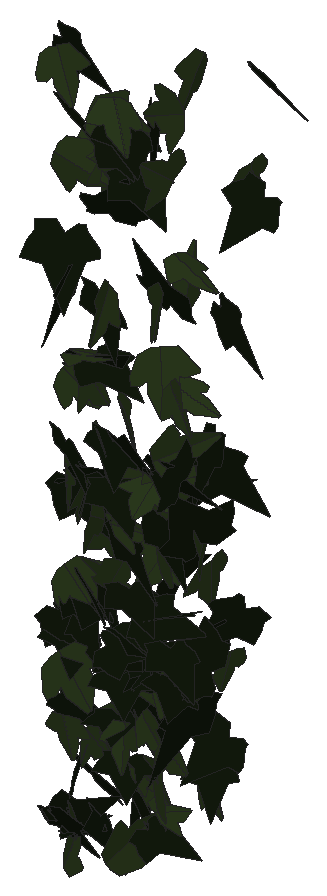
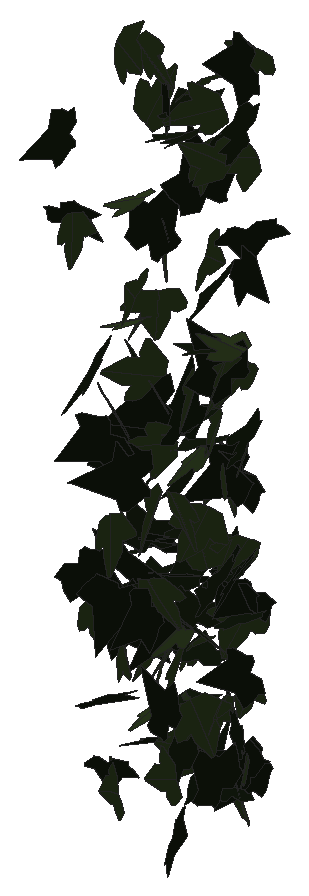
# SketchUp Ruby script. Lengths in inches.
U = 1.inch
M = Sketchup.active_model
def pt(a) = Geom::Point3d.new(a.map { |v| v * U })
def face(e, loops, mat)
  f = e.add_face(loops[0].map { |a| pt(a) })
  loops[1..].each { |l| e.add_face(l.map { |a| pt(a) }).erase! }
  f.material = f.back_material = mat if mat
  f
end
# faces: each face lists its corners as indices into pts; further lists are holes
def faces(e, pts, list, mat = nil) = list.each { |f| face(e, (f[0].is_a?(Array) ? f : [f]).map { |l| l.map { |i| pts[i] } }, mat) }
# xy, xz, yz: faces in a plane at the given z, y or x. An outline is a flat list of corners, or four numbers for a rectangle; further outlines are holes
def ring(l) = l.size == 4 ? [[l[0], l[1]], [l[2], l[1]], [l[2], l[3]], [l[0], l[3]]] : l.each_slice(2).to_a
def flat(e, list, mat, &to3) = list.each { |f| face(e, (f[0].is_a?(Array) ? f : [f]).map { |l| ring(l).map { |u, v| to3.(u, v) } }, mat) }
def xy(e, z, list, mat = nil) = flat(e, list, mat) { |x, y| [x, y, z] }
def xz(e, y, list, mat = nil) = flat(e, list, mat) { |x, z| [x, y, z] }
def yz(e, x, list, mat = nil) = flat(e, list, mat) { |y, z| [x, y, z] }
def lines(e, pts, list) = list.each { |a, b| e.add_line(pt(pts[a]), pt(pts[b])) }
# prism: a flat outline (further loops are holes) pulled along v
def prism(e, loops, v, mat = nil)
  f = face(e, loops, mat); d = Geom::Vector3d.new(v.map { |x| x * U })
  f.pushpull(f.normal.samedirection?(d) ? d.length : -d.length)
end
def box(e, o, s, mat = nil) = prism(e, [[o, [o[0] + s[0], o[1], o[2]], [o[0] + s[0], o[1] + s[1], o[2]], [o[0], o[1] + s[1], o[2]]]], [0, 0, s[2]], mat)
def at(x, y, z, deg = 0) = Geom::Transformation.translation(pt([x, y, z])) * Geom::Transformation.rotation(ORIGIN, Z_AXIS, deg.degrees)
def axes(o, x, y, z) = Geom::Transformation.new([*x, 0, *y, 0, *z, 0, *pt(o).to_a, 1])
def part(name) = M.definitions.add(name)
# library, detail: a bought-in or finely detailed component or shape, given as its bounding box
def library(name, o, s) = part(name).tap { |d| box(d.entities, o, s) }
def detail(e, o, s) = box(e.add_group.entities, o, s)
def put(e, d, t, mat = nil) = e.add_instance(d, t).tap { |i| i.material = mat if mat }
def group(e, t, mat = nil) = e.add_group.tap { |g| g.transformation = t; g.material = mat if mat }.entities
root = M.entities
M.materials.add("efeu1").color = [18, 25, 13]
M.materials.add("efeu2").color = [43, 57, 29]
c1 = part("ivyleaf_9")
p = [[1.54,2.16,1.25],[1.36,2.04,1.19],[-0.21,0.99,0.68],[-0.71,1.11,0.82],[-0.85,0.86,0.67],[-0.8,0.17,0.21],
  [-0.9,-0.01,0.1],[-0.67,-0.16,-0.02],[-0.08,-0.08,-0.05],[-0.03,-0.6,-0.4],[0.65,-0.88,-0.66],[0.83,-0.6,-0.49],
  [1.29,-0.42,-0.43],[1.8125,-0.07,-0.26],[1.21,0.44,0.15]]
faces(c1.entities,p,[[0,1,2,3,4,5,6,7,8,9,10,11,12,13,14]],"efeu1")
c2 = part("ivyleaf_10")
p = [[0,0.5,-0.03],[-0.0625,2.02,-0.43],[-0.19,2.01,-0.46],[-0.54,1.05,-0.29],[-0.52,0.625,-0.18],[-0.83,0.76,-0.28],
  [-1.16,0.64,-0.33],[-1.15,0.33,-0.24],[-0.77,-0.39,0.02],[-0.3,-0.51,0.16],[0.04,-0.48,0.23],[-0.02,2.01,-0.4375],
  [-0.06,2.01,-0.43],[0.04,-0.49,0.23],[0.67,-0.49,0.14],[1.38,0.36,-0.2],[1.375,0.51,-0.24],[0.81,0.65,-0.19],
  [0.62,0.59,-0.15],[0.6,1.09,-0.28],[0.5,1.23,-0.31]]
faces(c2.entities,p,[[0,1,2,3,4,5,6,7,8,9,10],[11,12,0,13,14,15,16,17,18,19,20]],"efeu2")
put(root,c1,axes([585.51,133.55,206.23],[0.0501,-0.05438,-1.04227],[0.86065,-0.58813,0.07206],[-0.5904,-0.86195,0.0166]))
put(root,c2,axes([585.95,127.96,211.29],[-0.83136,-0.03017,-0.08429],[0.08725,-0.09703,-0.82592],[0.02002,-0.82997,0.09962]))
put(root,c1,axes([585.42,128.3,216.13],[-0.09026,-0.32634,-0.83286],[0.52136,0.66101,-0.31551],[0.72686,-0.51465,0.12288]))
put(root,c2,axes([585.97,128.1,207.37],[-0.60504,0.54503,-0.03185],[0.01034,-0.03609,-0.81409],[-0.54586,-0.6048,0.01987]))
put(root,c1,axes([585.38,128.72,223.79],[0.42595,-0.76263,0.4513],[0.2309,-0.38792,-0.87346],[0.85555,0.48439,0.01104]))
put(root,c1,axes([585.28,128.95,239.36],[0.80558,-0.65014,0.25019],[0.21213,-0.13539,-1.03485],[0.66354,0.8326,0.02708]))
put(root,c1,axes([585.71,128.67,217.36],[0.49087,-0.72835,-0.41678],[-0.24025,0.34065,-0.87828],[0.80403,0.54645,-0.00799]))
put(root,c2,axes([585.78,128.51,227.15],[0.23963,0.72854,0.60869],[0.14768,0.59153,-0.76615],[-0.9378,0.27931,0.03489]))
put(root,c1,axes([585.8,128.06,233.9],[-0.38131,-0.98409,-0.33251],[0.16177,0.29362,-1.05452],[1.02607,-0.412,0.04269]))
put(root,c1,axes([585.67,128.77,214.84],[-0.23101,-0.84302,0.2977],[0.43214,-0.37446,-0.72505],[0.78266,-0.04207,0.48821]))
put(root,c2,axes([585.89,128.11,223.14],[-0.28014,0.63865,-0.5658],[0.20325,-0.52843,-0.6971],[-0.82868,-0.34551,0.02029]))
put(root,c1,axes([585.73,127.48,207.18],[0.96679,0.0946,-0.04957],[-0.04934,-0.00483,-0.97141],[-0.09472,0.96805,-0.00001]))
put(root,c1,axes([585.28,128.7,242.55],[0.21299,0.05407,-1.0631],[1.01754,0.30807,0.21953],[0.31262,-1.03954,0.00976]))
put(root,c1,axes([585.35,130.5,207.51],[0.24464,-0.58363,0.86638],[0.69801,-0.5707,-0.58154],[0.77719,0.69626,0.24958]))
put(root,c2,axes([586.21,128.98,222.03],[0.28492,-0.90487,-0.01439],[-0.00315,0.0141,-0.94866],[0.90498,0.28494,0.00123]))
put(root,c1,axes([585.48,128.43,212.1875],[0.11884,0.08634,-0.90899],[0.69514,0.5858,0.14653],[0.59204,-0.70515,0.01043]))
put(root,c1,axes([586.16,127.97,232.18],[-0.42791,0.42905,-0.87197],[0.63431,-0.5985,-0.60578],[-0.73625,-0.76501,-0.01511]))
put(root,c2,axes([585.98,128.12,204.92],[0.71411,-0.50695,-0.16028],[0.13019,-0.0935,0.87575],[-0.5155,-0.72588,-0.00086]))
put(root,c1,axes([585.99,128.37,208.41],[-0.04442,0.59072,0.69736],[0.04222,-0.69611,0.59235],[0.91295,0.06093,0.00654]))
put(root,c1,axes([585.72,128.72,222.29],[0.86826,0.29098,0.41673],[0.39648,0.12836,-0.91571],[-0.31801,0.95449,-0.0039]))
put(root,c2,axes([585.89,127.55,242.44],[0.86652,0.24684,0.42001],[0.40095,0.12548,-0.90094],[-0.27673,0.95473,0.00981]))
put(root,c2,axes([586.05,128.14,218.14],[0.3506,0.79192,0.47898],[0.19955,0.43547,-0.86604],[-0.90374,0.40338,-0.00541]))
put(root,c1,axes([585.67,128.7,222.19],[-0.13848,-0.22747,-1.05466],[0.8716,0.60312,-0.24453],[0.6359,-0.87621,0.10548]))
put(root,c2,axes([586.7,130.58,210.77],[-0.50125,-0.91522,0.38623],[-0.16473,-0.35004,-1.04326],[0.97963,-0.52716,0.02219]))
put(root,c1,axes([585.875,127.98,206.74],[0.09236,-0.0552,0.89328],[0.8896,0.104,-0.08555],[-0.09801,0.892,0.06525]))
put(root,c2,axes([586.33,128.9375,227.13],[0.23077,-0.84715,-0.50017],[0.28382,0.54923,-0.7993],[0.94195,0.04205,0.36337]))
put(root,c1,axes([586.02,128.57,216.49],[-0.32118,-0.34753,-0.79455],[0.69984,0.39652,-0.45633],[0.51216,-0.75976,0.12528]))
put(root,c2,axes([586.39,128.93,210.46],[0.20739,-0.73113,-0.50407],[0.25485,0.54486,-0.68544],[0.8507,0.01501,0.32823]))
put(root,c1,axes([585.88,130.07,217.07],[0.50797,-0.90302,0.37203],[0.18325,-0.32377,-1.03609],[0.95931,0.54001,0.00092]))
put(root,c2,axes([585.87,128.15,237.55],[-0.37364,-0.05689,-1.03887],[1.03345,-0.14794,-0.36359],[-0.12031,-1.09407,0.10319]))
put(root,c1,axes([586.04,128.92,206.21],[0.07892,-0.79624,0.09225],[0.78778,0.05993,-0.15666],[0.14801,0.10558,0.78465]))
put(root,c1,axes([585.93,129.24,227.16],[0.96059,0.40208,-0.31312],[0.29049,0.11694,1.04134],[0.41872,-1.00355,-0.00411]))
put(root,c1,axes([586.33,129.03,216.81],[-0.25324,-0.72445,0.51195],[0.3658,-0.57031,-0.62608],[0.80815,0.03113,0.44381]))
put(root,c2,axes([586.91,131.49,221.44],[0.88052,-0.45234,-0.39639],[-0.34182,0.20187,-0.98968],[0.49486,0.9443,0.02169]))
put(root,c2,axes([586.375,127.38,214.44],[0.58733,0.8968,0.53146],[0.18045,0.51333,-1.06564],[-1.02671,0.60323,0.11673]))
put(root,c2,axes([586.02,128.75,228.22],[0.02467,-0.91402,0.12488],[0.86123,0.06759,0.32456],[-0.3306,0.10787,0.85481]))
put(root,c2,axes([587.2,132.68,217.66],[0.95998,-0.05891,-0.44476],[-0.44464,0.01509,-0.96172],[0.05979,1.05789,-0.01105]))
put(root,c1,axes([586.38,128.84,217.4375],[0.29737,-0.59152,0.68094],[0.32778,-0.59711,-0.66184],[0.84032,0.44224,0.01719]))
put(root,c2,axes([586.49,129.02,237.47],[0.43719,0.37666,-0.93166],[0.7164,0.59568,0.57701],[0.70472,-0.83922,-0.00859]))
put(root,c2,axes([586.82,128.99,224.45],[-0.6376,0.84104,-0.32874],[0.19919,-0.26153,-1.05541],[-0.88077,-0.66799,-0.0007]))
put(root,c2,axes([587.04,129.67,219.86],[-0.85468,-0.48057,-0.40885],[0.34386,0.2224,-0.98024],[0.52902,-0.92096,-0.02338]))
put(root,c1,axes([587.45,132.85,216.65],[-0.12237,0.36293,-0.9901],[-0.57499,0.81257,0.36892],[0.88397,0.57879,0.10291]))
put(root,c1,axes([586.91,129.14,230.86],[0.30776,-0.96798,0.36038],[0.15468,-0.3286,-1.01473],[1.02124,0.34148,0.04509]))
put(root,c2,axes([587.62,127.62,221.7],[0.13548,-0.62675,-0.90074],[-0.01179,0.90669,-0.63266],[1.09727,0.08713,0.10441]))
put(root,c1,axes([586.77,128.98,228.12],[0.36483,-0.90552,-0.14975],[0.58802,0.35433,-0.71006],[0.70472,0.17313,0.66999]))
put(root,c2,axes([587.28,129.18,217.71],[-0.94553,-0.23681,0.48641],[0.48849,0.0472,0.97255],[-0.23249,1.06226,0.06522]))
put(root,c2,axes([587.48,129.02,237.49],[-0.02902,-1.00242,0.09044],[0.29754,-0.09498,-0.95724],[0.9615,-0.00086,0.29895]))
put(root,c1,axes([587.53,128.96,206.25],[0.80216,-0.78356,-0.41859],[0.29946,-0.29247,1.12135],[-0.83636,-0.85623,0.00003]))
put(root,c2,axes([587.86,129.36,225.93],[-0.70558,0.86897,-0.0138],[0.01865,-0.00263,-1.11928],[-0.86888,-0.70571,-0.01282]))
put(root,c2,axes([587.23,128.74,239.7],[0.26115,0.24354,1.04026],[0.74246,0.72867,-0.35699],[-0.76824,0.787,0.00861]))
put(root,c1,axes([587.5,129.07,224.36],[-0.02927,-0.84465,0.40291],[0.28462,-0.39204,-0.8012],[0.89149,0.09743,0.26903]))
put(root,c2,axes([587.19,131.6,207.68],[0.35692,-0.12655,0.97045],[0.97445,-0.04987,-0.3649],[0.09078,1.03281,0.10129]))
put(root,c1,axes([587.6,128.76,235.375],[1.04967,0.27832,0.13843],[-0.13377,-0.03564,1.08594],[0.2806,-1.05816,-0.00016]))
put(root,c1,axes([588.96,129.38,214.46],[-0.72522,0.63921,0.41019],[-0.50029,0.02469,-0.92298],[-0.57145,-0.83282,0.28747]))
put(root,c1,axes([587.53,130.44,207.62],[0.19374,-0.66892,0.82761],[0.38948,-0.73828,-0.68789],[0.99031,0.42122,0.10863]))
put(root,c2,axes([588.05,128.02,231.82],[-0.05489,0.68257,-0.8647],[0.0101,-0.86542,-0.68378],[-1.10159,-0.04195,0.03681]))
put(root,c1,axes([587.55,131.49,210.37],[0.03675,-0.09881,1.03993],[0.60851,-0.84377,-0.10168],[0.84908,0.60899,0.02785]))
put(root,c1,axes([587.82,129.05,214.26],[0.02158,-0.8249,0.21637],[0.81904,-0.04025,-0.23515],[0.2376,0.21368,0.79096]))
put(root,c1,axes([587.8,129.04,238.51],[0.35581,-0.93367,-0.1266],[0.37345,0.26399,-0.89734],[0.86505,0.27007,0.43946]))
put(root,c1,axes([588.11,128.61,212.09],[-0.37347,-0.77737,0.05048],[0.63513,-0.33627,-0.47944],[0.45106,-0.17015,0.71688]))
put(root,c1,axes([588.01,128.62,222.71],[-0.03244,-0.92644,-0.01219],[0.50749,-0.00756,-0.77582],[0.77518,-0.03382,0.5074]))
put(root,c2,axes([588.63,129.36,212.32],[-0.56231,0.99121,0.30142],[-0.15476,0.25875,-1.13958],[-1.0244,-0.58318,0.0067]))
put(root,c1,axes([588.25,128.81,213.9375],[-0.26663,-0.82743,-0.00445],[0.518,-0.16327,-0.6788],[0.64524,-0.21084,0.5431]))
put(root,c2,axes([588.21,128.35,240.48],[-0.43931,-0.87219,0.27213],[0.74852,-0.51672,-0.44774],[0.52391,0.0069,0.86789]))
put(root,c1,axes([588.4,129.35,223.71],[0.99687,-0.49364,-0.00519],[0.02825,0.04537,1.11112],[-0.49286,-0.99585,0.05319]))
put(root,c1,axes([588.37,128.87,209.99],[-0.25934,-0.8048,0.00532],[0.50405,-0.16678,-0.65811],[0.62743,-0.19867,0.53089]))
put(root,c1,axes([588.22,127.91,215.68],[0.69838,-0.36589,-0.36079],[0.31916,0.78599,-0.17928],[0.40272,0.0116,0.76777]))
put(root,c1,axes([588.39,128.8,239.3],[-0.0841,-0.99565,0.27704],[0.61092,-0.27209,-0.7924],[0.83358,0.09896,0.60869]))
put(root,c2,axes([588.71,129.03,213.47],[0.77089,-0.3383,-0.10328],[0.29825,0.75483,-0.2463],[0.19015,0.18754,0.80502]))
put(root,c2,axes([589.24,131.59,231.01],[-0.0105,0.68803,-0.80544],[-0.10541,0.8008,0.68544],[1.05404,0.08694,0.06052]))
put(root,c2,axes([588.81,127.73,221.51],[0.72353,-0.42561,-0.31545],[0.33095,0.78008,-0.29342],[0.41367,0.12033,0.78648]))
put(root,c2,axes([588.82,128.83,209.66],[0.63847,-0.52682,-0.16838],[0.37955,0.60441,-0.45185],[0.40228,0.26587,0.69355]))
put(root,c1,axes([589.03,129.21,214.02],[0.09104,-0.15727,-1.03371],[-0.33118,0.97986,-0.17825],[0.99178,0.34164,0.03537]))
put(root,c2,axes([588.95,127.9,211.93],[-0.19522,-0.71494,0.40095],[0.459,-0.43683,-0.55543],[0.67913,0.08973,0.49065]))
put(root,c1,axes([588.89,128.8125,215.63],[-0.35953,-0.54045,0.59252],[0.45125,-0.67312,-0.34015],[0.66297,0.16508,0.55285]))
put(root,c2,axes([589.59,129.8,219.73],[-0.34118,0.54893,1.02714],[-0.59501,0.83792,-0.64544],[-1.00115,-0.68506,0.03357]))
put(root,c2,axes([589.22,127.34,206.6],[0.03048,-0.65193,1.0668],[-0.04023,1.06606,0.65262],[-1.24958,-0.05022,0.00501]))
put(root,c1,axes([588.75,128.64,218.13],[0.10596,-0.8889,0.0101],[0.49677,0.05078,-0.74304],[0.7372,0.09355,0.49925]))
put(root,c1,axes([588.82,128,221.1],[0.71758,-0.84416,-0.05188],[-0.03637,0.03717,-1.10793],[0.84497,0.7185,-0.00363]))
put(root,c2,axes([588.68,133.58,207.37],[0.38025,-0.22211,1.01301],[0.97021,-0.30496,-0.43105],[0.36636,1.03816,0.0901]))
put(root,c2,axes([589.49,129.08,222.93],[-0.83499,-0.23028,0.23547],[0.23395,-0.86639,-0.0177],[0.23182,0.0449,0.86598]))
put(root,c1,axes([589.18,134.18,228.86],[0.80041,-0.67234,-0.4119],[-0.30019,0.2829,-1.04509],[0.7291,0.85457,0.0219]))
put(root,c1,axes([589.51,133.11,208.33],[-0.49372,-0.50572,-0.39636],[0.31205,0.24823,-0.70542],[0.56167,-0.58245,0.0435]))
put(root,c1,axes([589.3,129.3,238.82],[-0.02262,0.20015,1.06889],[0.22127,-1.04591,0.20053],[1.06472,0.22161,-0.01896]))
put(root,c1,axes([589.15,128.54,237.67],[0.11771,-0.97751,-0.1594],[0.54974,0.19801,-0.80831],[0.82384,0.00754,0.56215]))
put(root,c1,axes([589.19,131.43,221.88],[0.60487,0.17213,0.85059],[0.76513,0.38347,-0.6217],[-0.40951,0.97073,0.09477]))
put(root,c2,axes([589.5,128.68,212.22],[0.24395,-0.81519,-0.05507],[0.51489,0.19801,-0.65019],[0.63439,0.15276,0.5489]))
put(root,c2,axes([589.34,129.43,222.64],[-0.03915,0.00827,-1.09935],[0.8295,0.72216,-0.0241],[0.72151,-0.82981,-0.03194]))
put(root,c2,axes([590.69,130.73,212.6],[-0.07073,0.03834,1.06216],[-0.93652,0.50111,-0.08045],[-0.50258,-0.93919,0.00043]))
put(root,c1,axes([589.54,129.55,221.39],[0.53482,-0.95946,-0.06539],[-0.03152,0.0573,-1.09845],[0.96116,0.53575,0.00037]))
put(root,c2,axes([590.15,134.73,235.59],[-0.11309,-0.91447,-0.21238],[0.06287,0.20606,-0.92073],[0.9367,-0.12424,0.03616]))
put(root,c1,axes([590.58,128.875,232.12],[0.79019,-0.61193,0.69678],[-0.5583,0.41701,0.99938],[-0.74044,-0.96747,-0.00995]))
put(root,c1,axes([589.68,128.58,217.27],[0.57418,-0.43182,-0.55746],[0.39776,0.79194,-0.20378],[0.58225,-0.11517,0.68893]))
put(root,c2,axes([590.2,128.77,229.28],[0.74838,0.87208,0.04465],[0.0312,0.03207,-1.14917],[-0.87266,0.74903,-0.00279]))
put(root,c2,axes([591.08,128.52,241.23],[0.46293,-0.31074,-0.97167],[-0.83341,0.50017,-0.55701],[0.58833,0.95304,-0.02448]))
put(root,c2,axes([590.58,128.11,232.45],[0.76217,-0.8197,-0.34255],[-0.11156,0.35946,-1.10837],[0.88136,0.75434,0.15593]))
put(root,c1,axes([589.91,128.53,207.42],[0.45195,-0.54444,-0.42315],[0.34386,0.6165,-0.42594],[0.59769,0.057,0.56503]))
put(root,c1,axes([590.66,131.02,215.58],[0.36378,0.97962,0.1096],[0.05947,0.0948,-1.04474],[-0.98394,0.36791,-0.02263]))
put(root,c2,axes([591.11,127.76,209.14],[-0.31278,0.61221,-0.90819],[-0.39431,0.81822,0.68736],[1.02182,0.50314,-0.01275]))
put(root,c2,axes([590.82,131.24,218.78],[-0.0716,-1.03514,-0.23916],[0.04525,0.23651,-1.03723],[1.06145,-0.07991,0.02808]))
put(root,c1,axes([589.98,128.77,224.11],[0.9529,-0.09324,0.45213],[0.45039,-0.03986,-0.95744],[0.10133,1.05397,0.00379]))
put(root,c2,axes([590.63,130.62,242.39],[0.18395,-0.86556,0.7367],[0.33027,-0.67338,-0.87363],[1.08758,0.35088,0.1407]))
put(root,c2,axes([590.89,128.45,238.22],[-0.19094,-0.65608,-0.90815],[-0.22412,-0.88026,0.68305],[-1.0977,0.29385,0.01851]))
put(root,c2,axes([590.65,128.29,208.59],[0.70855,-0.24216,-0.35179],[0.22335,0.79095,-0.09461],[0.36402,-0.01394,0.74279]))
put(root,c1,axes([590.97,132.11,210.5],[-0.69962,-0.64794,0.3322],[0.00374,-0.46388,-0.89691],[0.72813,-0.62019,0.3238]))
put(root,c1,axes([590.33,134.97,240.1],[0.89038,-0.34202,0.15946],[0.15989,-0.02821,-0.95332],[0.34182,0.90411,0.03058]))
put(root,c1,axes([590.37,129.11,217.32],[0.02104,-0.80491,0.3292],[0.85345,-0.0441,-0.16237],[0.16693,0.32691,0.78864]))
put(root,c2,axes([590.82,128.35,211.64],[0.09128,-0.77363,-0.38003],[0.3752,0.37972,-0.68286],[0.77598,-0.0926,0.37488]))
put(root,c2,axes([590.77,128.33,214.46],[0.23149,-0.74732,-0.4149],[0.4994,0.4671,-0.5627],[0.69371,-0.08688,0.54354]))
put(root,c2,axes([590.8125,128.49,225.14],[-0.07012,-0.37064,1.08543],[0.32453,1.03661,0.37493],[-1.10009,0.32942,0.04142]))
put(root,c1,axes([591.14,131.08,224.87],[-0.77094,0.02008,-0.65434],[0.64561,-0.14409,-0.76508],[-0.10841,-1.00087,0.09701]))
put(root,c2,axes([591.49,131.64,214.67],[-0.25621,-0.79966,0.09892],[-0.04098,-0.09073,-0.83962],[0.80471,-0.25922,-0.01126]))
put(root,c1,axes([591.65,133.55,235.27],[-0.84741,-0.43025,0.01467],[-0.02077,0.00852,-0.95023],[0.43,-0.8475,-0.017]))
put(root,c1,axes([592.12,127.54,224.84],[-0.518,0.71169,0.61535],[-0.35748,0.50089,-0.88023],[-0.87027,-0.62936,-0.0047]))
put(root,c1,axes([590.73,131.59,223.53],[-0.06287,-0.11772,-1.07569],[0.74692,0.77493,-0.12846],[0.78299,-0.74869,0.03617]))
put(root,c2,axes([591.76,129.33,220.75],[0.1142,-0.05359,-1.06829],[-0.29797,1.03024,-0.08353],[1.02729,0.30479,0.09453]))
put(root,c1,axes([591.92,131.98,216.85],[-0.0175,0.22308,-0.94051],[-0.14664,-0.93039,-0.21795],[-0.95542,0.13871,0.05068]))
put(root,c1,axes([591.74,129.03,213.59],[-0.34431,0.66889,-1.08885],[0.49587,-0.96939,-0.7523],[-1.17776,-0.60368,0.00158]))
put(root,c1,axes([591.71,129.51,221.125],[0.55931,0.35477,1.03144],[-0.86869,-0.55611,0.66233],[0.65963,-1.03317,-0.00233]))
put(root,c1,axes([591.27,128.33,214.64],[-0.25273,-0.75707,0.37184],[0.40335,-0.4494,-0.64081],[0.74076,-0.01359,0.4758]))
put(root,c2,axes([591.27,128.24,228.34],[0.25468,-0.92799,0.02656],[0.55279,0.12946,-0.77743],[0.74585,0.22092,0.56712]))
put(root,c1,axes([592.67,128.82,215.72],[-0.63728,0.38851,0.94094],[-0.81385,0.47241,-0.74627],[-0.61152,-1.0336,0.0126]))
put(root,c1,axes([591.16,128.3,216.34],[0.09624,-0.88216,-0.09627],[0.39325,0.1292,-0.79082],[0.7955,0.04285,0.40258]))
put(root,c2,axes([591.03,129.12,228.05],[0.02337,-0.89415,-0.23749],[0.90487,0.07156,-0.1804],[0.19266,-0.22765,0.87607]))
put(root,c2,axes([591.05,129.11,234.01],[0.02483,-0.94995,0.09036],[0.93511,0.00621,-0.19164],[0.19013,0.0935,0.93075]))
